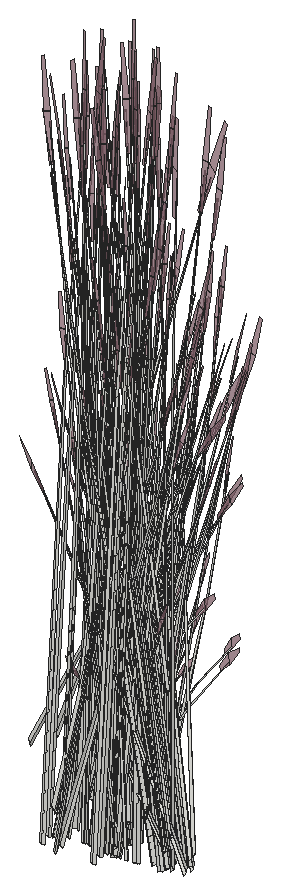
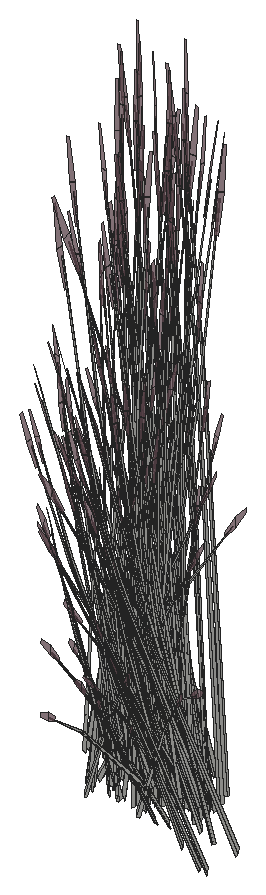
# SketchUp Ruby script. Lengths in inches.
U = 1.inch
M = Sketchup.active_model
def pt(a) = Geom::Point3d.new(a.map { |v| v * U })
def face(e, loops, mat)
  f = e.add_face(loops[0].map { |a| pt(a) })
  loops[1..].each { |l| e.add_face(l.map { |a| pt(a) }).erase! }
  f.material = f.back_material = mat if mat
  f
end
# faces: each face lists its corners as indices into pts; further lists are holes
def faces(e, pts, list, mat = nil) = list.each { |f| face(e, (f[0].is_a?(Array) ? f : [f]).map { |l| l.map { |i| pts[i] } }, mat) }
# xy, xz, yz: faces in a plane at the given z, y or x. An outline is a flat list of corners, or four numbers for a rectangle; further outlines are holes
def ring(l) = l.size == 4 ? [[l[0], l[1]], [l[2], l[1]], [l[2], l[3]], [l[0], l[3]]] : l.each_slice(2).to_a
def flat(e, list, mat, &to3) = list.each { |f| face(e, (f[0].is_a?(Array) ? f : [f]).map { |l| ring(l).map { |u, v| to3.(u, v) } }, mat) }
def xy(e, z, list, mat = nil) = flat(e, list, mat) { |x, y| [x, y, z] }
def xz(e, y, list, mat = nil) = flat(e, list, mat) { |x, z| [x, y, z] }
def yz(e, x, list, mat = nil) = flat(e, list, mat) { |y, z| [x, y, z] }
def lines(e, pts, list) = list.each { |a, b| e.add_line(pt(pts[a]), pt(pts[b])) }
# prism: a flat outline (further loops are holes) pulled along v
def prism(e, loops, v, mat = nil)
  f = face(e, loops, mat); d = Geom::Vector3d.new(v.map { |x| x * U })
  f.pushpull(f.normal.samedirection?(d) ? d.length : -d.length)
end
def box(e, o, s, mat = nil) = prism(e, [[o, [o[0] + s[0], o[1], o[2]], [o[0] + s[0], o[1] + s[1], o[2]], [o[0], o[1] + s[1], o[2]]]], [0, 0, s[2]], mat)
def at(x, y, z, deg = 0) = Geom::Transformation.translation(pt([x, y, z])) * Geom::Transformation.rotation(ORIGIN, Z_AXIS, deg.degrees)
def axes(o, x, y, z) = Geom::Transformation.new([*x, 0, *y, 0, *z, 0, *pt(o).to_a, 1])
def part(name) = M.definitions.add(name)
# library, detail: a bought-in or finely detailed component or shape, given as its bounding box
def library(name, o, s) = part(name).tap { |d| box(d.entities, o, s) }
def detail(e, o, s) = box(e.add_group.entities, o, s)
def put(e, d, t, mat = nil) = e.add_instance(d, t).tap { |i| i.material = mat if mat }
def group(e, t, mat = nil) = e.add_group.tap { |g| g.transformation = t; g.material = mat if mat }.entities
root = M.entities
M.materials.add("LightPink_Translucent").color = [144, 107, 117]
M.materials["LightPink_Translucent"].alpha = 0.75
c1 = part("blade")
p = [[2.15,0.21,22],[0,0.17,0],[0.09,0.45,0],[2.18,0.31,22],[2.29,0.31,22],[0.38,0.45,0],
  [2.48,0.24,33],[2.49,0.24,33],[2.48,0.22,33]]
faces(c1.entities,p,[[0,1,2,3],[4,5,2,3],[6,3,4,7],[8,0,3,6]])
c2 = part("seeds")
p = [[0.3,-0.1,1.38],[-0.01,-0.03,1.59],[-0.01,-0.03,0.03],[0.14,-0.07,-0.07],[0.29,-0.03,3],[0.15,0.01,3.11]]
faces(c2.entities,p,[[0,1,2,3],[1,0,4,5]],"LightPink_Translucent")
c3 = part("blade with seeds")
put(c3.entities,c1,at(0,0,0))
put(c3.entities,c2,axes([2.4,0.25,30.99],[1.5799,-0.05474,1.17369],[-0.12525,1.92788,0.29478],[-0.07173,-0.02425,1.56792]))
put(root,c3,axes([664.71,345.73,391.24],[-0.034,-0.08668,1.46364],[0.23582,-0.50706,-0.2236],[0.23788,-0.00729,0.24931]))
put(root,c3,axes([667.41,342.26,394.13],[0.31051,0.46426,-0.58968],[-0.63919,0.25873,0.07116],[0.07261,0.22432,0.83415]))
put(root,c3,axes([670.68,340.6,391.83],[-0.81312,-0.00457,-0.0413],[0,-0.63814,0.41452],[-0.02555,0.14527,1.31432]))
put(root,c3,axes([664.93,347.92,393.91],[-0.05883,-0.04999,1.47228],[0.12868,-0.53581,-0.13912],[0.23172,-0.03423,0.26054]))
put(root,c3,axes([672.55,342.4,391.67],[-0.60889,0.28548,-0.4121],[-0.36394,-0.51192,0],[-0.13868,0.06502,1.30728]))
put(root,c3,axes([672.45,342.43,391.24],[0.08727,0.05704,1.46364],[0.14797,0.52853,-0.2236],[-0.19341,0.11271,0.24931]))
put(root,c3,axes([662.5,345.6,393.22],[-0.26985,0.01293,1.42242],[0.17902,-0.56047,0.11501],[0.38456,0.03467,0.60807]))
put(root,c3,axes([672.59,342.25,391.82],[-0.40169,-0.57414,-0.04268],[0.68052,-0.31907,0.42834],[-0.16769,0.05466,1.35813]))
put(root,c3,axes([669.08,338.68,392.05],[-0.6991,0.15154,0.14643],[-0.17263,-0.56398,0.29122],[0.06235,0.08217,1.33138]))
put(root,c3,axes([670.01,341.99,394.15],[0.46573,0.38364,-0.47077],[-0.49199,0.33598,-0.36465],[-0.07086,0.19492,0.90078]))
put(root,c3,axes([668.0625,343.76,394.6875],[0.44958,-0.32756,-0.05385],[0.41194,0.35875,-0.24415],[0.029,0.10165,0.8053]))
put(root,c3,axes([672.41,342.17,391.68],[-0.60696,-0.14127,-0.25712],[0.15283,-0.49751,0.25712],[-0.12236,0.05737,1.15348]))
put(root,c3,axes([672.84,340.95,393.93],[-0.16135,-0.52549,0.39842],[0.63294,-0.0912,0.32852],[-0.18654,0.12359,0.82444]))
put(root,c3,axes([663.49,346.13,394.13],[0.57168,-0.25217,-0.58968],[0.3186,0.51908,0.07116],[0.27622,-0.05897,0.83415]))
put(root,c3,axes([669.81,341.7,394.19],[0.4402,-0.30062,0.29394],[0.41671,0.34326,-0.37948],[-0.0634,0.1744,0.72609]))
put(root,c3,axes([668.86,340.32,391.84],[0.45414,0.3688,0],[-0.45414,0.3688,0],[0,0,1.40491]))
put(root,c3,axes([668.86,339.89,392.26],[0.31565,-0.51449,0.37133],[0.65588,0.24761,-0.17871],[0,0.1186,1.19224]))
put(root,c3,axes([672.76,340.04,392.36],[-0.01777,-0.53759,1.17256],[0.80434,0.13935,0.49647],[-0.19024,0.29416,1.1068]))
put(root,c3,axes([668.58,341.68,391.83],[0.65588,0.25634,0],[-0.31565,0.53263,0],[0,0,1.45212]))
put(root,c3,axes([672.71,340.85,393.93],[-0.44663,-0.24013,0.05337],[0.26003,-0.34195,0.42015],[-0.14319,0.11055,0.64067]))
put(root,c3,axes([667.65,342.36,393.89],[0.63954,0.14313,-0.42412],[-0.21921,0.49074,-0.32852],[0.05864,0.19758,0.81151]))
put(root,c3,axes([667.1,342.38,394.18],[0.63664,-0.26583,-0.10093],[0.31286,0.47181,-0.56021],[0.084,0.19882,0.85122]))
put(root,c3,axes([665.41,345.58,393.91],[0.09028,-0.08697,1.45204],[-0.11555,-0.53348,-0.22964],[0.22652,-0.10115,0.11645]))
put(root,c3,axes([669.53,341.78,394.48],[0.71502,0.02829,-0.11203],[-0.01954,0.53563,-0.62183],[-0.04967,0.20629,0.94486]))
put(root,c3,axes([668.64,339.77,391.98],[-0.82229,-0.1203,0.40835],[0.16734,-0.67942,0.16024],[0.12017,0.06561,1.41775]))
put(root,c3,axes([669.51,342.5625,392.34],[0.59102,-0.10111,0.05401],[0.13587,0.40735,-0.71633],[-0.03747,0.2062,0.64209]))
put(root,c3,axes([672.3,340.73,392.21],[0.07581,0.65151,-0.24149],[-0.7896,0.03939,-0.41502],[-0.13904,0.08678,1.32557]))
put(root,c3,axes([673.62,341.02,393.22],[0.12114,-0.19625,1.42242],[0.50818,0.40613,0.11501],[-0.22925,0.25313,0.60807]))
put(root,c3,axes([670.51,340.7,391.68],[-0.45414,0.35624,-0.25712],[-0.45414,-0.35624,0.25712],[0,0.11474,1.15348]))
put(root,c3,axes([670.54,341.44,393.22],[-0.01592,-0.21915,1.42242],[0.69015,0.14538,0.11501],[-0.04269,0.3123,0.60807]))
put(root,c3,axes([669.21,340.63,391.74],[0.23855,0.52277,-0.57446],[-0.68718,0.18827,-0.15077],[0.02637,0.17702,1.26801]))
put(root,c3,axes([664.37,346.9,392.15],[-0.15668,-0.14043,1.18691],[0.20386,-0.46454,-0.25526],[0.31701,0.06293,0.50747]))
put(root,c3,axes([668.88,340.07,391.83],[0.72788,0,0],[0,0.59111,0],[0,0,1.48078]))
put(root,c3,axes([673.13,339.66,394.19],[0.54068,0.15928,0.29394],[-0.1577,0.46469,-0.37948],[-0.21769,0.04261,0.72609]))
put(root,c3,axes([669.13,340.01,392.17],[0.60616,-0.16651,0.12018],[0.21227,0.47548,-0.34318],[0,0.10465,1.05198]))
put(root,c3,axes([673.23,341.1,393.89],[0.16713,0.52135,-0.42412],[-0.63294,0.0912,-0.32852],[-0.18138,0.14003,0.81151]))
put(root,c3,axes([672.24,342.04,393.91],[-0.01617,0.11299,1.45204],[0.45894,0.39307,-0.22964],[-0.12015,0.18588,0.11645]))
put(root,c3,axes([668.92,340.05,392.21],[0.73268,0.27244,-0.24149],[-0.35279,0.57501,-0.41502],[0.02303,0.14118,1.32557]))
put(root,c3,axes([672.93,340.73,394.18],[0.60181,0.31483,-0.10093],[-0.34671,0.45593,-0.56021],[-0.17003,0.15849,0.85122]))
put(root,c3,axes([670.51,340.18,392.06],[0,-0.57097,0.4121],[0.72788,0,0],[0,0.13004,1.30728]))
put(root,c3,axes([670.82,340.71,391.67],[0,0.57097,-0.4121],[-0.72788,0,0],[0,0.13004,1.30728]))
put(root,c3,axes([668.88,342.4375,393.93],[-0.64708,0.13103,0.39842],[-0.1123,-0.514,0.32852],[0.15218,0.15149,0.82444]))
put(root,c3,axes([671.59,341.67,391.82],[-0.65588,-0.25634,0],[0.31565,-0.53263,0],[0,0,1.35047]))
put(root,c3,axes([668.76,342.54,393.93],[-0.29569,0.36271,0.05337],[-0.42107,-0.21117,0.42015],[0.13613,0.11629,0.64067]))
put(root,c3,axes([673.1,342.31,391.97],[0.40676,0.57214,0],[-0.68052,0.31907,-0.42834],[-0.15499,0.07267,1.3588]))
put(root,c3,axes([668.01,341.34,393.22],[-0.14872,-0.18332,1.42242],[0.6872,-0.15433,0.11501],[0.15531,0.28779,0.60807]))
put(root,c3,axes([674.29,342.17,391.97],[-0.40676,0.57214,0],[-0.68052,-0.31907,-0.42834],[-0.15499,-0.07267,1.3588]))
put(root,c3,axes([671.03,342.56,394.2],[-0.64106,-0.14927,0.44225],[0.21921,-0.49074,0.36465],[0.03852,0.19299,0.91512]))
put(root,c3,axes([676.98,340.21,393.22],[0.22574,-0.12077,1.42242],[0.19004,0.55807,0.11501],[-0.35439,0.12613,0.60807]))
put(root,c3,axes([670.86,342.59,393.93],[-0.47939,0.19405,0.05337],[-0.23464,-0.35385,0.42015],[0.0463,0.15598,0.64067]))
put(root,c3,axes([672.77,341.61,392.05],[0.18794,-0.56744,0.14643],[0.68774,0.16058,0.29122],[-0.1188,0.00276,1.33138]))
put(root,c3,axes([671.9375,342.1,394.6875],[0.5741,0.15241,-0.05385],[-0.1766,0.46909,-0.24415],[-0.0939,0.07122,0.8053]))
put(root,c3,axes([672.45,340.86,392.17],[0.48065,0.34305,0.12018],[-0.40092,0.38703,-0.34318],[-0.1116,0.05232,1.05198]))
put(root,c3,axes([676.28,341.16,392.15],[0.2261,0.04687,1.18691],[0.14573,0.47875,-0.25526],[-0.30712,0.08962,0.50747]))
put(root,c3,axes([673.22,340.77,394.19],[0.56631,-0.0816,0.29394],[0.14954,0.46647,-0.37948],[-0.16229,0.12529,0.72609]))
put(root,c3,axes([672.4375,340.6,392.26],[0.70648,-0.03525,0.37133],[0.06389,0.58508,-0.17871],[-0.12647,0.0593,1.19224]))
put(root,c3,axes([668.78,341.375,391.8125],[0.68303,-0.19373,-0.15934],[0.24001,0.55805,0.00007],[0.07539,-0.02141,1.44335]))
put(root,c3,axes([673.55,342.99,392.15],[0.2053,-0.09007,1.18691],[0.50689,0.27159,-0.25526],[-0.15087,0.235,0.50747]))
put(root,c3,axes([672.61,341.95,391.93],[0.81449,0.18558,0.25528],[-0.20377,0.66335,-0.30288],[-0.13481,0.08302,1.36855]))
put(root,c3,axes([678.28,339.63,392.77],[0.18493,-0.0826,1.46963],[0.06377,0.5767,0.11501],[-0.40056,0.07652,0.52526]))
put(root,c3,axes([672.96,341.91,392.06],[0.60889,-0.28548,0.4121],[0.36394,0.51192,0],[-0.13868,0.06502,1.30728]))
put(root,c3,axes([668.67,342.12,394.19],[-0.10048,-0.4599,0.29394],[0.5744,-0.12144,-0.37948],[0.15428,0.13179,0.72609]))
put(root,c3,axes([668.79,339.72,391.83],[0.39083,0.47924,-0.37133],[-0.59199,0.33747,0.17871],[0.12647,0.0593,1.19224]))
put(root,c3,axes([671.74,341.45,391.83],[-0.21227,-0.49226,0],[0.60616,-0.17239,0],[0,0,1.28128]))
put(root,c3,axes([670.96,342.48,391.24],[0.10529,-0.03107,1.46364],[0.63335,0.17101,-0.2236],[0.01852,0.19274,0.24931]))
put(root,c3,axes([675.58,340.8125,392.21],[-0.65687,0.37907,-0.24149],[-0.43681,-0.53562,-0.41502],[-0.16207,-0.0544,1.32557]))
put(root,c3,axes([673.76,342.01,393.93],[-0.46327,-0.38957,0.39842],[0.49199,-0.33598,0.32852],[-0.08546,0.18277,0.82444]))
put(root,c3,axes([669.05,339.48,393.71],[-0.56218,-0.29666,1.14775],[0.59361,-0.46189,0.49522],[0.18138,0.27836,1.10941]))
put(root,c3,axes([671.1,342.66,393.76],[-0.19614,0.43908,-0.29394],[-0.57222,-0.12807,0.37948],[0.05247,0.17678,0.72609]))
put(root,c3,axes([668.11,342.77,393.91],[0.00193,-0.06913,1.47228],[0.55753,-0.30498,-0.13912],[0.19366,0.10886,0.26054]))
put(root,c3,axes([676.29,340.02,393.91],[-0.10624,0.07413,1.45204],[0.00904,0.54162,-0.22964],[-0.24352,0.07044,0.11645]))
put(root,c3,axes([669.9,341.89,392.3],[-0.36631,-0.16417,0.95334],[0.47299,-0.16681,0.70045],[0.12758,0.1413,0.20998]))
put(root,c3,axes([668.6,341.72,392.15],[0.01148,-0.18927,1.18691],[0.54864,-0.21141,-0.25526],[0.16937,0.22654,0.50747]))
put(root,c3,axes([673.59,341.97,393.93],[-0.53464,-0.0266,0.05337],[0.01466,-0.40172,0.42015],[-0.05594,0.15388,0.64067]))
put(root,c3,axes([673.76,342.13,393.76],[-0.4402,0.30062,-0.29394],[-0.41671,-0.34326,0.37948],[-0.0634,0.1744,0.72609]))
put(root,c3,axes([672.59,340.48,391.83],[-0.31565,0.51449,-0.37133],[-0.65588,-0.24761,0.17871],[0,0.1186,1.19224]))
put(root,c3,axes([676.01,341.23,391.71],[-0.43821,0.42916,-0.51753],[-0.54436,-0.38915,-0.13583],[-0.1756,0.10706,1.14236]))
put(root,c3,axes([672.1875,343.2,393.91],[0.07381,-0.03447,1.47228],[0.61004,0.22929,-0.13912],[-0.01434,0.19091,0.26054]))
put(root,c3,axes([670.7,343.4375,393.91],[0.08247,0.09194,1.45204],[0.66552,0.03612,-0.22964],[0.06692,0.20277,0.11645]))
put(root,c3,axes([669.86,338.65,391.68],[0.15283,0.49751,-0.25712],[-0.60696,0.14127,0.25712],[0.12236,0.05737,1.15348]))
put(root,c3,axes([671.01,340.28,391.97],[0.81352,0,0],[0,0.63814,-0.42834],[0,0.14534,1.3588]))
put(root,c3,axes([673.84,340.16,392.05],[-0.51116,-0.4159,0.14643],[0.51512,-0.4034,0.29122],[-0.05645,0.08494,1.33138]))
put(root,c3,axes([675.11,340.5625,393.91],[0.08303,0.01531,1.47228],[0.25685,0.50448,-0.13912],[-0.16996,0.13241,0.26054]))
put(root,c3,axes([677,339.94,393.89],[-0.17625,0.51936,-0.42412],[-0.60429,-0.17802,-0.32852],[-0.2433,0.04762,0.81151]))
put(root,c3,axes([672.48,340.19,391.9],[0,0.66033,-0.04679],[-0.81352,0,0],[0,0.02075,1.48875]))
put(root,c3,axes([671.04,342.2,394.19],[0.19614,-0.43908,0.29394],[0.57222,0.12807,-0.37948],[0.05247,0.17678,0.72609]))
put(root,c3,axes([669.96,342.64,392.21],[-0.4172,-0.01791,0.872],[0.27552,-0.38032,0.48145],[0.16481,0.13512,0.68401]))
put(root,c3,axes([676.3125,340.99,392.05],[-0.63528,-0.45956,-0.20909],[0.53456,-0.51604,0.45758],[-0.17107,0.05376,1.39619]))
put(root,c3,axes([672.09,341.46,391.9],[0.28286,0.65594,-0.0499],[-0.80821,0.22985,0],[0.00988,0.02291,1.42904]))
put(root,c3,axes([674.05,341.81,394.43],[-0.01693,0.52814,-0.65454],[-0.71285,-0.03547,0.07899],[-0.07523,0.22375,0.92591]))
put(root,c3,axes([674.04,343.3,392.3],[-0.01684,-0.3395,0.95334],[0.42072,0.24214,0.70045],[-0.08274,0.16182,0.20998]))
put(root,c3,axes([675.99,340.89,391.83],[-0.70648,0.03525,-0.37133],[-0.06389,-0.58508,0.17871],[-0.12647,0.0593,1.19224]))
put(root,c3,axes([675.81,342.17,392.3],[0.27113,-0.25877,0.95334],[0.10699,0.40966,0.70045],[-0.19594,0.07335,0.20998]))
put(root,c3,axes([671.16,342.26,394.13],[0.31051,0.46426,-0.58968],[-0.63919,0.25873,0.07116],[0.07261,0.22432,0.83415]))
put(root,c3,axes([674.43,340.6,391.83],[-0.81312,-0.00457,-0.0413],[0,-0.63814,0.41452],[-0.02555,0.14527,1.31432]))
put(root,c3,axes([668.61,342.36,394.18],[0.38768,-0.48872,-0.10093],[0.56143,0.28156,-0.56021],[0.19516,0.13808,0.85122]))
put(root,c3,axes([676.98,339.5,394.18],[0.32734,0.51701,-0.10093],[-0.58097,0.25407,-0.56021],[-0.24483,0.06821,0.85122]))
put(root,c3,axes([672.83,338.68,392.05],[-0.6991,0.15154,0.14643],[-0.17263,-0.56398,0.29122],[0.06235,0.08217,1.33138]))
put(root,c3,axes([674.64,341.87,392.06],[0.60889,0.28548,0.4121],[-0.36394,0.51192,0],[-0.13868,-0.06502,1.30728]))
put(root,c3,axes([673.8125,342.55,392.79],[0.01429,-0.29475,1.28107],[0.64291,0.15569,0.17703],[-0.0557,0.31414,0.60492]))
put(root,c3,axes([677.81,340.59,393.22],[0.1625,-0.17544,1.42242],[0.41029,0.47354,0.11501],[-0.28141,0.21565,0.60807]))
put(root,c3,axes([676.83,341.05,393.76],[-0.56631,0.0816,-0.29394],[-0.14954,-0.46647,0.37948],[-0.16229,0.12529,0.72609]))
put(root,c3,axes([671.8125,343.76,394.6875],[0.44958,-0.32756,-0.05385],[0.41194,0.35875,-0.24415],[0.029,0.10165,0.8053]))
put(root,c3,axes([669.07,342.12,393.89],[0.64198,-0.13573,-0.42412],[0.1123,0.514,-0.32852],[0.17243,0.1473,0.81151]))
put(root,c3,axes([672.61,340.32,391.84],[0.45414,0.3688,0],[-0.45414,0.3688,0],[0,0,1.40491]))
put(root,c3,axes([676.52,342.43,391.24],[0.08727,0.05704,1.46364],[0.14797,0.52853,-0.2236],[-0.19341,0.11271,0.24931]))
put(root,c3,axes([675.51,340.98,392.17],[-0.12551,0.50956,0.12018],[-0.6132,-0.08845,-0.34318],[-0.1116,-0.05232,1.05198]))
put(root,c3,axes([672.6,339.89,392.26],[0.31565,-0.51449,0.37133],[0.65588,0.24761,-0.17871],[0,0.1186,1.19224]))
put(root,c3,axes([672.33,341.68,391.83],[0.65588,0.25634,0],[-0.31565,0.53263,0],[0,0,1.45212]))
put(root,c3,axes([669.81,341.5,394.19],[-0.37017,-0.35748,0.29394],[0.42268,-0.3384,-0.37948],[0.21476,0.05149,0.72609]))
put(root,c3,axes([676.73,342.4,391.67],[-0.60889,0.28548,-0.4121],[-0.36394,-0.51192,0],[-0.13868,0.06502,1.30728]))
put(root,c3,axes([676.77,342.25,391.82],[-0.40169,-0.57414,-0.04268],[0.68052,-0.31907,0.42834],[-0.16769,0.05466,1.35813]))
put(root,c3,axes([671.4,342.36,393.89],[0.63954,0.14313,-0.42412],[-0.21921,0.49074,-0.32852],[0.05864,0.19758,0.81151]))
put(root,c3,axes([670.85,342.38,394.18],[0.63664,-0.26583,-0.10093],[0.31286,0.47181,-0.56021],[0.084,0.19882,0.85122]))
put(root,c3,axes([672.39,339.77,391.98],[-0.82229,-0.1203,0.40835],[0.16734,-0.67942,0.16024],[0.12017,0.06561,1.41775]))
put(root,c3,axes([676.9,340.95,393.93],[-0.16135,-0.52549,0.39842],[0.63294,-0.0912,0.32852],[-0.18654,0.12359,0.82444]))
put(root,c3,axes([670.15,341.83,393.93],[-0.03276,0.43418,0.05337],[-0.49468,-0.0119,0.42015],[0.18949,0.04543,0.64067]))
put(root,c3,axes([670,342.5,391.24],[0.0474,-0.08243,1.46364],[0.59674,-0.24277,-0.2236],[0.18092,0.12565,0.24931]))
put(root,c3,axes([674.2,341.99,394.15],[0.46573,0.38364,-0.47077],[-0.49199,0.33598,-0.36465],[-0.07086,0.19492,0.90078]))
put(root,c3,axes([670.19,341.6875,393.93],[-0.47971,0.37622,0.39842],[-0.41372,-0.39954,0.32852],[0.22506,0.0694,0.82444]))
put(root,c3,axes([674.26,340.7,391.68],[-0.45414,0.35624,-0.25712],[-0.45414,-0.35624,0.25712],[0,0.11474,1.15348]))
put(root,c3,axes([676.59,342.17,391.68],[-0.60696,-0.14127,-0.25712],[0.15283,-0.49751,0.25712],[-0.12236,0.05737,1.15348]))
put(root,c3,axes([673.99,341.7,394.19],[0.4402,-0.30062,0.29394],[0.41671,0.34326,-0.37948],[-0.0634,0.1744,0.72609]))
put(root,c3,axes([676.78,340.85,393.93],[-0.44663,-0.24013,0.05337],[0.26003,-0.34195,0.42015],[-0.14319,0.11055,0.64067]))
put(root,c3,axes([671.4375,341.74,393.26],[-0.12452,-0.47997,-0.02898],[0.58854,-0.11034,-0.1314],[0.1229,0.03043,0.43341]))
put(root,c3,axes([676.9375,340.04,392.36],[-0.01777,-0.53759,1.17256],[0.80434,0.13935,0.49647],[-0.19024,0.29416,1.1068]))
put(root,c3,axes([672.96,340.63,391.74],[0.23855,0.52277,-0.57446],[-0.68718,0.18827,-0.15077],[0.02637,0.17702,1.26801]))
put(root,c3,axes([672.625,340.07,391.83],[0.72788,0,0],[0,0.59111,0],[0,0,1.48078]))
put(root,c3,axes([669.15,339.53,391.71],[0.67676,0.09361,-0.51753],[-0.14281,0.57742,-0.13583],[0.20196,0.06997,1.14236]))
put(root,c3,axes([672.88,340.01,392.17],[0.60616,-0.16651,0.12018],[0.21227,0.47548,-0.34318],[0,0.10465,1.05198]))
put(root,c3,axes([677.6875,341.02,393.22],[0.12114,-0.19625,1.42242],[0.50818,0.40613,0.11501],[-0.22925,0.25313,0.60807]))
put(root,c3,axes([673.71,341.78,394.48],[0.71502,0.02829,-0.11203],[-0.01954,0.53563,-0.62183],[-0.04967,0.20629,0.94486]))
put(root,c3,axes([673.69,342.5625,392.34],[0.59102,-0.10111,0.05401],[0.13587,0.40735,-0.71633],[-0.03747,0.2062,0.64209]))
put(root,c3,axes([676.49,340.73,392.21],[0.07581,0.65151,-0.24149],[-0.7896,0.03939,-0.41502],[-0.13904,0.08678,1.32557]))
put(root,c3,axes([677.2,339.66,394.19],[0.54068,0.15928,0.29394],[-0.1577,0.46469,-0.37948],[-0.21769,0.04261,0.72609]))
put(root,c3,axes([672.67,340.05,392.21],[0.73268,0.27244,-0.24149],[-0.35279,0.57501,-0.41502],[0.02303,0.14118,1.32557]))
